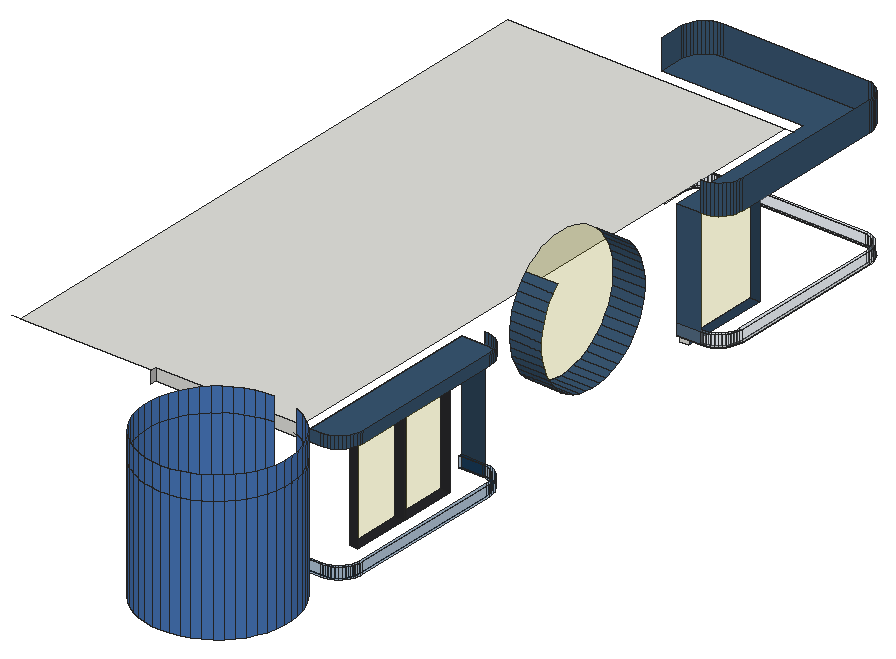
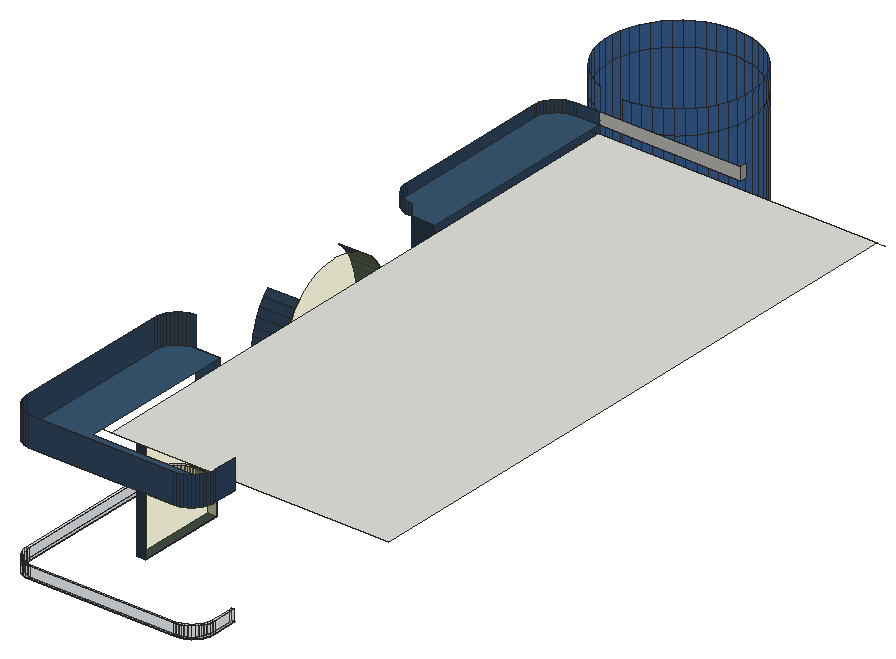
# SketchUp Ruby script. Lengths in inches.
U = 1.inch
M = Sketchup.active_model
def pt(a) = Geom::Point3d.new(a.map { |v| v * U })
def face(e, loops, mat)
  f = e.add_face(loops[0].map { |a| pt(a) })
  loops[1..].each { |l| e.add_face(l.map { |a| pt(a) }).erase! }
  f.material = f.back_material = mat if mat
  f
end
# faces: each face lists its corners as indices into pts; further lists are holes
def faces(e, pts, list, mat = nil) = list.each { |f| face(e, (f[0].is_a?(Array) ? f : [f]).map { |l| l.map { |i| pts[i] } }, mat) }
# xy, xz, yz: faces in a plane at the given z, y or x. An outline is a flat list of corners, or four numbers for a rectangle; further outlines are holes
def ring(l) = l.size == 4 ? [[l[0], l[1]], [l[2], l[1]], [l[2], l[3]], [l[0], l[3]]] : l.each_slice(2).to_a
def flat(e, list, mat, &to3) = list.each { |f| face(e, (f[0].is_a?(Array) ? f : [f]).map { |l| ring(l).map { |u, v| to3.(u, v) } }, mat) }
def xy(e, z, list, mat = nil) = flat(e, list, mat) { |x, y| [x, y, z] }
def xz(e, y, list, mat = nil) = flat(e, list, mat) { |x, z| [x, y, z] }
def yz(e, x, list, mat = nil) = flat(e, list, mat) { |y, z| [x, y, z] }
def lines(e, pts, list) = list.each { |a, b| e.add_line(pt(pts[a]), pt(pts[b])) }
# prism: a flat outline (further loops are holes) pulled along v
def prism(e, loops, v, mat = nil)
  f = face(e, loops, mat); d = Geom::Vector3d.new(v.map { |x| x * U })
  f.pushpull(f.normal.samedirection?(d) ? d.length : -d.length)
end
def box(e, o, s, mat = nil) = prism(e, [[o, [o[0] + s[0], o[1], o[2]], [o[0] + s[0], o[1] + s[1], o[2]], [o[0], o[1] + s[1], o[2]]]], [0, 0, s[2]], mat)
def at(x, y, z, deg = 0) = Geom::Transformation.translation(pt([x, y, z])) * Geom::Transformation.rotation(ORIGIN, Z_AXIS, deg.degrees)
def axes(o, x, y, z) = Geom::Transformation.new([*x, 0, *y, 0, *z, 0, *pt(o).to_a, 1])
def part(name) = M.definitions.add(name)
# library, detail: a bought-in or finely detailed component or shape, given as its bounding box
def library(name, o, s) = part(name).tap { |d| box(d.entities, o, s) }
def detail(e, o, s) = box(e.add_group.entities, o, s)
def put(e, d, t, mat = nil) = e.add_instance(d, t).tap { |i| i.material = mat if mat }
def group(e, t, mat = nil) = e.add_group.tap { |g| g.transformation = t; g.material = mat if mat }.entities
root = M.entities
M.materials.add("Carpet_01_1K").color = [196, 195, 193]
M.materials.add("Carpet_04_1K").color = [56, 85, 112]
M.materials.add("Carpet_04_1K1").color = [43, 65, 85]
M.materials.add("Glass_Basic_01").color = [186, 175, 28]
M.materials["Glass_Basic_01"].alpha = 0.25
M.materials.add("Glass_Basic_1").color = [0, 47, 91]
M.materials["Glass_Basic_1"].alpha = 0.25
M.materials.add("Glass_Basic_2").color = [161, 173, 186]
M.materials["Glass_Basic_2"].alpha = 0.25
M.materials.add("Glass_Mirror_01").color = [71, 118, 185]
M.materials.add("ThomThom - Buttons2").color = [40, 40, 43]
c1 = part("Group\#1")
prism(c1.entities,[[[0,206.04,0],[0,209.04,0],[24,209.04,0],[24.001,209.04,0],[27.133,208.835,0],[30.212,208.222,0],[33.184,207.213,0],[36,205.825,0],[38.61,204.081,0],[40.971,202.011,0],[43.04,199.65,0],[44.785,197.04,0],[46.173,194.224,0],[47.182,191.252,0],[47.795,188.173,0],[48,185.04,0],[48,24,0],[47.795,20.867,0],[47.182,17.788,0],[46.602,16.08,0],[46.173,14.816,0],[44.785,12,0],[43.04,9.39,0],[40.971,7.029,0],[38.61,4.96,0],[36,3.215,0],[33.184,1.827,0],[30.212,0.818,0],[27.133,0.205,0],[24,0,0],[0,0,0],[0,3,0],[3,3,0],[24,3,0],[26.741,3.18,0],[29.435,3.716,0],[32.036,4.599,0],[34.5,5.814,0],[36.784,7.34,0],[38.849,9.151,0],[40.66,11.216,0],[42.187,13.5,0],[43.401,15.964,0],[44.284,18.565,0],[44.82,21.259,0],[45,24,0],[45,185.04,0],[44.82,187.781,0],[44.284,190.475,0],[43.401,193.076,0],[42.187,195.54,0],[40.66,197.824,0],[38.849,199.889,0],[36.784,201.701,0],[34.5,203.227,0],[32.036,204.442,0],[29.435,205.325,0],[26.741,205.86,0],[24,206.04,0],[3,206.04,0]]],[0,0,12])
c2 = part("Group\#2")
prism(c2.entities,[[[147,3,0],[168,3,0],[170.74,3.18,0],[173.44,3.72,0],[176.04,4.6,0],[178.5,5.8125,0],[180.78,7.34,0],[182.85,9.15,0],[184.66,11.22,0],[186.1875,13.5,0],[187.4,15.96,0],[188.28,18.56,0],[188.82,21.26,0],[189,24,0],[189,184.94,0],[188.8125,187.78,0],[188.28,190.47,0],[187.4,193.07,0],[186.18,195.54,0],[184.66,197.82,0],[182.84,199.88,0],[180.78,201.7,0],[178.5,203.22,0],[176.03,204.4375,0],[173.43,205.32,0],[171.01,205.8,0],[24,205.8,0],[21.26,205.62,0],[18.56,205.08,0],[15.96,204.2,0],[13.5,202.99,0],[11.22,201.46,0],[9.15,199.65,0],[7.34,197.58,0],[5.8125,195.3,0],[4.6,192.84,0],[3.72,190.24,0],[3.18,187.54,0],[3,184.8,0],[3,163.8,0],[3,160.8,0],[0,160.8,0],[0,184.8,0],[0.21,187.93,0],[0.82,191.01,0],[1.83,193.98,0],[3.22,196.8,0],[4.96,199.41,0],[7.03,201.77,0],[9.39,203.84,0],[12,205.58,0],[14.82,206.97,0],[17.79,207.98,0],[20.87,208.59,0],[24,208.8,0],[171.31,208.8,0],[174.21,208.22,0],[177.18,207.21,0],[180,205.82,0],[182.61,204.08,0],[184.97,202.01,0],[187.04,199.65,0],[188.78,197.04,0],[190.17,194.22,0],[191.18,191.25,0],[191.79,188.17,0],[192,185.04,0],[192,24,0],[191.79,20.87,0],[191.18,17.79,0],[190.17,14.82,0],[188.78,12,0],[187.04,9.39,0],[184.97,7.03,0],[182.61,4.96,0],[180,3.22,0],[177.18,1.83,0],[174.21,0.82,0],[171.13,0.21,0],[168,0,0],[144,0,0],[144,3,0]]],[0,0,12])
xy(root,314,[[321.57,233.15,330.57,291.15],[321.57,293.15,330.57,349.15]],"ThomThom - Buttons2")
xy(root,315,[[321.57,652.9,330.57,742.9]],"Carpet_04_1K1")
xy(root,330,[[330.57,637.9,354.57,637.9,357.71,638.11,360.79,638.72,363.76,639.73,366.57,641.12,369.19,642.86,371.55,644.93,373.62,647.29,375.36,649.9,376.75,652.72,377.76,655.6875,378.37,658.77,378.57,661.9,378.57,822.94,378.37,826.07,377.76,829.15,376.75,832.125,375.36,834.94,373.62,837.55,371.55,839.91,369.19,841.98,366.57,843.73,363.76,845.11,360.79,846.12,357.88,846.7,210.57,846.7,207.44,846.5,204.36,845.88,201.39,844.875,198.57,843.49,195.96,841.74,193.6,839.67,191.53,837.3125,189.79,834.7,188.4,831.89,187.39,828.91,186.78,825.83,186.57,822.7,186.57,798.7,189.57,798.7,189.57,822.7,189.75,825.44,190.29,828.14,191.17,830.74,192.39,833.2,193.91,835.48,195.73,837.55,197.79,839.36,200.07,840.89,202.54,842.1,205.14,842.99,207.83,843.52,210.57,843.7,357.59,843.7,360.01,843.22,362.61,842.34,365.07,841.12,367.36,839.6,369.42,837.79,371.23,835.72,372.76,833.4375,373.97,830.97,374.85,828.375,375.39,825.68,375.57,822.84,375.57,661.9,375.4,659.16,374.86,656.47,373.98,653.86,372.76,651.4,371.24,649.12,369.42,647.05,367.36,645.24,365.07,643.71,362.61,642.5,360.01,641.62,357.32,641.08,354.57,640.9,330.57,640.9]])
xy(root,429,[[321.57,652.9,330.57,742.9]],"Carpet_04_1K1")
xy(root,436,[[321.57,233.15,330.57,291.15],[321.57,293.15,330.57,349.15]])
xy(root,450,[[39.57,167.5625,321.57,786.64]])
xy(root,450,[[330.57,155.5,330.57,364.54,354.58,364.54,357.71,364.34,360.79,363.72,363.76,362.71,366.57,361.33,369.19,359.58,371.55,357.51,373.62,355.15,375.36,352.54,376.75,349.73,377.76,346.75,378.37,343.67,378.57,340.54,378.57,179.5,378.37,176.37,377.76,173.29,376.75,170.32,375.36,167.5,373.62,164.89,371.55,162.53,369.19,160.46,366.57,158.72,363.76,157.33,360.79,156.32,357.71,155.71,354.57,155.5],[330.57,637.9,330.57,798.7,186.57,798.7,186.57,822.7,186.78,825.83,187.39,828.91,188.4,831.89,189.79,834.7,191.53,837.3125,193.6,839.67,195.96,841.74,198.57,843.49,201.39,844.875,204.36,845.88,207.44,846.5,210.57,846.7,357.88,846.7,360.79,846.12,363.76,845.11,366.57,843.73,369.19,841.98,371.55,839.91,373.62,837.55,375.36,834.94,376.75,832.125,377.76,829.15,378.37,826.07,378.57,822.94,378.57,661.9,378.37,658.77,377.76,655.6875,376.75,652.72,375.36,649.9,373.62,647.29,371.55,644.93,369.19,642.86,366.57,641.12,363.76,639.73,360.79,638.72,357.71,638.11,354.57,637.9]],"Carpet_04_1K")
xz(root,155.5,[[186.57,450,330.57,462]])
xz(root,155.5,[[330.57,450,354.57,461.77]],"Carpet_04_1K")
xz(root,233.15,[[321.57,314,330.57,436]],"ThomThom - Buttons2")
xz(root,291.15,[[321.57,314,330.57,436]],"ThomThom - Buttons2")
xz(root,293.15,[[321.57,314,330.57,436]],"ThomThom - Buttons2")
xz(root,349.15,[[321.57,314,330.57,436]],"ThomThom - Buttons2")
xz(root,364.54,[[354.57,450,354.58,461.77]])
xz(root,364.54,[[330.57,330,354.57,438],[330.57,438,354.57,450]],"Carpet_04_1K1")
xz(root,435.35,[[322.57,412.91,354.57,421.2]],"Carpet_04_1K")
xz(root,567.09,[[322.57,412.8,354.57,421.09]],"Carpet_04_1K")
xz(root,637.9,[[330.57,330,354.57,450]],"Carpet_04_1K")
xz(root,652.9,[[321.57,315,330.57,429]])
xz(root,742.9,[[321.57,315,330.57,429]],"Carpet_04_1K1")
xz(root,846.7,[[210.57,450,357.88,480]],"Carpet_04_1K")
yz(root,186.57,[[149.51,450,155.5,462]],"Carpet_01_1K")
yz(root,186.57,[[798.7,450,822.7,480]],"Carpet_04_1K")
yz(root,236.92,[[77.22,330,86.26,456],[77.22,456,86.26,480]],"Glass_Mirror_01")
yz(root,321.57,[[233.15,314,291.15,436],[293.15,314,349.15,436],[652.9,315,742.9,429]],"Glass_Basic_01")
yz(root,322.57,[[501.17,351,509.44,351.51,517.58,353.0625,525.47,355.62,532.97,359.14,539.97,363.57,546.36,368.85,552.04,374.89,556.92,381.59,560.92,388.85,563.97,396.56,566.04,404.58,567.09,412.8,567.09,421.09,566.0625,429.32,564.01,437.35,560.96,445.05,556.97,452.32,552.11,459.03,546.4375,465.08,540.06,470.36,533.0625,474.8125,525.57,478.35,517.68,480.91,509.54,482.47,501.27,483,501.22,483,493,482.49,484.86,480.9375,476.97,478.38,469.47,474.86,462.47,470.43,456.08,465.15,450.4,459.11,445.52,452.41,441.52,445.15,438.47,437.44,436.4,429.42,435.35,421.2,435.35,412.91,436.38,404.68,438.44,396.65,441.48,388.95,445.47,381.68,450.33,374.97,456,368.92,462.39,363.64,469.38,359.1875,476.875,355.65,484.76,353.09,492.9,351.53]],"Glass_Basic_01")
yz(root,330.57,[[155.5,438,364.54,450]],"Carpet_04_1K")
yz(root,378.57,[[179.5,450,340.54,461.77],[661.9,450,822.94,480]],"Carpet_04_1K")
yz(root,380.64,[[77.22,330,86.26,456],[77.22,456,86.26,480]],"Glass_Mirror_01")
p = [[299.76,10.31,456],[299.76,10.3,330],[308.78,9.74,330],[308.78,9.74,456],[317.8,10.3,330],[317.8,10.31,456],
  [290.875,12,456],[290.875,12,330],[326.6875,12,330],[326.6875,12,456],[282.28,14.79,456],[282.28,14.79,330],
  [335.29,14.79,330],[335.29,14.79,456],[274.09,18.64,456],[274.09,18.64,330],[343.47,18.64,330],[343.47,18.64,456],
  [266.46,23.49,456],[266.46,23.49,330],[351.1,23.49,330],[351.1,23.49,456],[259.49,29.25,456],[259.49,29.25,330],
  [358.07,29.25,330],[358.07,29.25,456],[253.3,35.84,456],[253.3,35.84,330],[364.26,35.84,330],[364.26,35.84,456],
  [247.99,43.16,456],[247.99,43.16,330],[369.57,43.16,330],[369.57,43.16,456],[243.63,51.08,456],[243.63,51.08,330],
  [373.93,51.08,330],[373.93,51.08,456],[240.3,59.49,456],[240.3,59.49,330],[377.26,59.49,330],[377.26,59.49,456],
  [238.06,68.25,456],[238.06,68.25,330],[379.51,68.25,330],[379.51,68.25,456],[236.92,77.22,456],[236.92,77.22,330],
  [380.64,77.22,330],[380.64,77.22,456],[238.06,95.23,456],[238.06,95.23,330],[236.92,86.26,330],[236.92,86.26,456],
  [380.64,86.26,456],[380.64,86.26,330],[379.51,95.23,330],[379.51,95.23,456],[240.3,103.99,456],[240.3,103.99,330],
  [377.26,103.99,330],[377.26,103.99,456],[243.63,112.39,456],[243.63,112.39,330],[373.93,112.39,330],[373.93,112.39,456],
  [247.99,120.32,456],[247.99,120.32,330],[369.57,120.32,330],[369.57,120.32,456],[253.3,127.63,456],[253.3,127.63,330],
  [364.26,127.63,330],[364.26,127.63,456],[259.49,134.22,456],[259.49,134.22,330],[358.07,134.22,330],[358.07,134.22,456],
  [266.46,139.99,456],[266.46,139.99,330],[351.1,139.99,330],[351.1,139.99,456],[274.09,144.83,456],[274.09,144.83,330],
  [343.47,144.83,330],[343.47,144.83,456],[282.28,148.68,456],[282.28,148.68,330],[335.29,148.68,330],[335.29,148.68,456],
  [290.875,151.48,456],[290.875,151.48,330],[299.76,153.17,456],[299.76,153.17,330],[308.78,153.74,456],[308.78,153.74,330],
  [322.57,492.9,351.53],[354.57,492.9,351.53],[354.57,501.17,351],[322.57,501.17,351],[354.57,509.44,351.51],[322.57,509.44,351.51],
  [322.57,484.76,353.09],[354.57,484.76,353.09],[354.57,517.58,353.0625],[322.57,517.58,353.0625],[322.57,476.875,355.65],[354.57,476.875,355.65],
  [354.57,525.47,355.62],[322.57,525.47,355.62],[354.57,532.97,359.14],[322.57,532.97,359.14],[322.57,469.38,359.1875],[354.57,469.38,359.1875],
  [354.57,539.97,363.57],[322.57,539.97,363.57],[322.57,462.39,363.64],[354.57,462.39,363.64],[322.57,456,368.92],[354.57,456,368.92],
  [354.57,546.36,368.85],[322.57,546.36,368.85],[322.57,450.33,374.97],[354.57,450.33,374.97],[354.57,552.04,374.89],[322.57,552.04,374.89],
  [354.57,556.92,381.59],[322.57,556.92,381.59],[322.57,445.47,381.68],[354.57,445.47,381.68],[354.57,560.92,388.85],[322.57,560.92,388.85],
  [322.57,441.48,388.95],[354.57,441.48,388.95],[322.57,438.44,396.65],[354.57,438.44,396.65],[354.57,563.97,396.56],[322.57,563.97,396.56],
  [354.57,566.04,404.58],[322.57,566.04,404.58],[322.57,436.38,404.68],[354.57,436.38,404.68],[354.57,567.09,412.8],[322.57,567.09,412.8],
  [322.57,435.35,412.91],[354.57,435.35,412.91],[322.57,567.09,421.09],[354.57,567.09,421.09],[354.57,566.0625,429.32],[322.57,566.0625,429.32],
  [322.57,436.4,429.42],[354.57,436.4,429.42],[354.57,435.35,421.2],[322.57,435.35,421.2],[354.57,564.01,437.35],[322.57,564.01,437.35],
  [322.57,438.47,437.44],[354.57,438.47,437.44],[354.57,560.96,445.05],[322.57,560.96,445.05],[322.57,441.52,445.15],[354.57,441.52,445.15],
  [322.57,445.52,452.41],[354.57,445.52,452.41],[354.57,556.97,452.32],[322.57,556.97,452.32],[357.71,155.71,450],[357.71,155.71,461.77],
  [354.57,155.5,461.77],[354.57,155.5,450],[360.79,156.32,450],[360.79,156.32,461.77],[363.76,157.33,450],[363.76,157.33,461.77],
  [366.57,158.72,450],[366.57,158.72,461.77],[369.19,160.46,450],[369.19,160.46,461.77],[371.55,162.53,450],[371.55,162.53,461.77],
  [373.62,164.89,450],[373.62,164.89,461.77],[375.36,167.5,450],[375.36,167.5,461.77],[376.75,170.32,450],[376.75,170.32,461.77],
  [377.76,173.29,450],[377.76,173.29,461.77],[378.37,176.37,450],[378.37,176.37,461.77],[378.57,179.5,450],[378.57,179.5,461.77],
  [378.37,343.67,450],[378.37,343.67,461.77],[378.57,340.54,461.77],[378.57,340.54,450],[377.76,346.75,450],[377.76,346.75,461.77],
  [376.75,349.73,450],[376.75,349.73,461.77],[375.36,352.54,450],[375.36,352.54,461.77],[373.62,355.15,450],[373.62,355.15,461.77],
  [371.55,357.51,450],[371.55,357.51,461.77],[369.19,359.58,450],[369.19,359.58,461.77],[366.57,361.33,450],[366.57,361.33,461.77],
  [363.76,362.71,450],[363.76,362.71,461.77],[360.79,363.72,450],[360.79,363.72,461.77],[357.71,364.34,450],[357.71,364.34,461.77],
  [354.58,364.54,450],[354.58,364.54,461.77],[357.71,638.11,450],[357.71,638.11,480],[354.57,637.9,480],[354.57,637.9,450],
  [360.79,638.72,450],[360.79,638.72,480],[363.76,639.73,450],[363.76,639.73,480],[366.57,641.12,450],[366.57,641.12,480],
  [369.19,642.86,450],[369.19,642.86,480],[371.55,644.93,450],[371.55,644.93,480],[373.62,647.29,450],[373.62,647.29,480],
  [375.36,649.9,450],[375.36,649.9,480],[376.75,652.72,450],[376.75,652.72,480],[377.76,655.6875,450],[377.76,655.6875,480],
  [378.37,658.77,450],[378.37,658.77,480],[378.57,661.9,450],[378.57,661.9,480],[186.57,822.7,450],[186.57,822.7,480],
  [186.78,825.83,480],[186.78,825.83,450],[378.37,826.07,450],[378.37,826.07,480],[378.57,822.94,480],[378.57,822.94,450],
  [187.39,828.91,480],[187.39,828.91,450],[377.76,829.15,450],[377.76,829.15,480],[188.4,831.89,480],[188.4,831.89,450],
  [376.75,832.125,450],[376.75,832.125,480],[189.79,834.7,480],[189.79,834.7,450],[375.36,834.94,450],[375.36,834.94,480],
  [191.53,837.3125,480],[191.53,837.3125,450],[373.62,837.55,450],[373.62,837.55,480],[193.6,839.67,480],[193.6,839.67,450],
  [371.55,839.91,450],[371.55,839.91,480],[195.96,841.74,480],[195.96,841.74,450],[369.19,841.98,450],[369.19,841.98,480],
  [198.57,843.49,480],[198.57,843.49,450],[366.57,843.73,450],[366.57,843.73,480],[201.39,844.875,480],[201.39,844.875,450],
  [363.76,845.11,450],[363.76,845.11,480],[204.36,845.88,480],[204.36,845.88,450],[360.79,846.12,450],[360.79,846.12,480],
  [207.44,846.5,480],[207.44,846.5,450],[357.88,846.7,462],[357.88,846.7,480],[357.88,846.7,450],[210.57,846.7,480],
  [210.57,846.7,450],[354.57,552.11,459.03],[322.57,552.11,459.03],[322.57,450.4,459.11],[354.57,450.4,459.11],[308.78,9.74,480],
  [299.76,10.31,480],[317.8,10.31,480],[290.875,12,480],[326.6875,12,480],[282.28,14.79,480],[335.29,14.79,480],
  [274.09,18.64,480],[343.47,18.64,480],[266.46,23.49,480],[351.1,23.49,480],[259.49,29.25,480],[358.07,29.25,480],
  [253.3,35.84,480],[364.26,35.84,480],[247.99,43.16,480],[369.57,43.16,480],[243.63,51.08,480],[373.93,51.08,480],
  [240.3,59.49,480],[377.26,59.49,480],[238.06,68.25,480],[379.51,68.25,480],[236.92,77.22,480],[380.64,77.22,480],
  [236.92,86.26,480],[238.06,95.23,480],[379.51,95.23,480],[380.64,86.26,480],[240.3,103.99,480],[377.26,103.99,480],
  [243.63,112.39,480],[373.93,112.39,480],[247.99,120.32,480],[369.57,120.32,480],[253.3,127.63,480],[364.26,127.63,480],
  [259.49,134.22,480],[358.07,134.22,480],[266.46,139.99,480],[351.1,139.99,480],[274.09,144.83,480],[343.47,144.83,480],
  [282.28,148.68,480],[335.29,148.68,480],[290.875,151.48,480],[299.76,153.17,480],[308.78,153.74,480],[354.57,546.4375,465.08],
  [322.57,546.4375,465.08],[322.57,456.08,465.15],[354.57,456.08,465.15],[39.57,167.5625,450],[30.57,167.5625,450],[321.57,167.5625,450],
  [330.57,167.5625,450],[321.57,786.64,450],[330.57,786.64,450],[330.57,150.21,456],[330.57,150.21,330]]
faces(root,p,[[0,1,2,3],[3,2,4,5],[6,7,1,0],[5,4,8,9],[10,11,7,6],[9,8,12,13],[14,15,11,10],[13,12,16,17],
  [18,19,15,14],[17,16,20,21],[22,23,19,18],[21,20,24,25],[26,27,23,22],[25,24,28,29],[30,31,27,26],[29,28,32,33],
  [34,35,31,30],[33,32,36,37],[38,39,35,34],[37,36,40,41],[42,43,39,38],[41,40,44,45],[46,47,43,42],[45,44,48,49],
  [50,51,52,53],[54,55,56,57],[58,59,51,50],[57,56,60,61],[62,63,59,58],[61,60,64,65],[66,67,63,62],[65,64,68,69],
  [70,71,67,66],[69,68,72,73],[74,75,71,70],[73,72,76,77],[78,79,75,74],[77,76,80,81],[82,83,79,78],[81,80,84,85],
  [86,87,83,82],[85,84,88,89],[90,91,87,86],[92,93,91,90],[94,95,93,92],[3,299,300,0],[5,301,299,3],[0,300,302,6],
  [9,303,301,5],[6,302,304,10],[13,305,303,9],[10,304,306,14],[17,307,305,13],[14,306,308,18],[21,309,307,17],[18,308,310,22],
  [25,311,309,21],[22,310,312,26],[29,313,311,25],[26,312,314,30],[33,315,313,29],[30,314,316,34],[37,317,315,33],[34,316,318,38],
  [41,319,317,37],[38,318,320,42],[45,321,319,41],[42,320,322,46],[49,323,321,45],[53,324,325,50],[57,326,327,54],[50,325,328,58],
  [61,329,326,57],[58,328,330,62],[65,331,329,61],[62,330,332,66],[69,333,331,65],[66,332,334,70],[73,335,333,69],[70,334,336,74],
  [77,337,335,73],[74,336,338,78],[81,339,337,77],[78,338,340,82],[85,341,339,81],[82,340,342,86],[89,343,341,85],[86,342,344,90],
  [90,344,345,92],[92,345,346,94]],"Glass_Mirror_01")
faces(root,p,[[96,97,98,99],[99,98,100,101],[102,103,97,96],[101,100,104,105],[106,107,103,102],[105,104,108,109],[109,108,110,111],[112,113,107,106],
  [111,110,114,115],[116,117,113,112],[118,119,117,116],[115,114,120,121],[122,123,119,118],[121,120,124,125],[125,124,126,127],[128,129,123,122],
  [127,126,130,131],[132,133,129,128],[134,135,133,132],[131,130,136,137],[137,136,138,139],[140,141,135,134],[139,138,142,143],[144,145,141,140],
  [146,147,148,149],[150,151,152,153],[149,148,154,155],[156,157,151,150],[155,154,158,159],[160,161,157,156],[162,163,161,160],[159,158,164,165],
  [166,167,168,169],[170,171,167,166],[172,173,171,170],[174,175,173,172],[176,177,175,174],[178,179,177,176],[180,181,179,178],[182,183,181,180],
  [184,185,183,182],[186,187,185,184],[188,189,187,186],[190,191,189,188],[192,193,194,195],[196,197,193,192],[198,199,197,196],[200,201,199,198],
  [202,203,201,200],[204,205,203,202],[206,207,205,204],[208,209,207,206],[210,211,209,208],[212,213,211,210],[214,215,213,212],[216,217,215,214],
  [218,219,220,221],[222,223,219,218],[224,225,223,222],[226,227,225,224],[228,229,227,226],[230,231,229,228],[232,233,231,230],[234,235,233,232],
  [236,237,235,234],[238,239,237,236],[240,241,239,238],[242,243,241,240],[244,245,246,247],[248,249,250,251],[247,246,252,253],[254,255,249,248],
  [253,252,256,257],[258,259,255,254],[257,256,260,261],[262,263,259,258],[261,260,264,265],[266,267,263,262],[265,264,268,269],[270,271,267,266],
  [269,268,272,273],[274,275,271,270],[273,272,276,277],[278,279,275,274],[277,276,280,281],[282,283,279,278],[281,280,284,285],[286,287,283,282],
  [285,284,288,289],[290,291,287,286,292],[289,288,293,294],[165,164,295,296],[297,298,163,162],[296,295,347,348],[349,350,298,297]],"Carpet_04_1K")
lines(root,p,[[351,352],[353,354],[355,356],[89,357],[88,358]])
put(root,c1,at(330.57,155.5,330),"Glass_Basic_1")
put(root,c2,at(186.57,637.9,330),"Glass_Basic_2")
